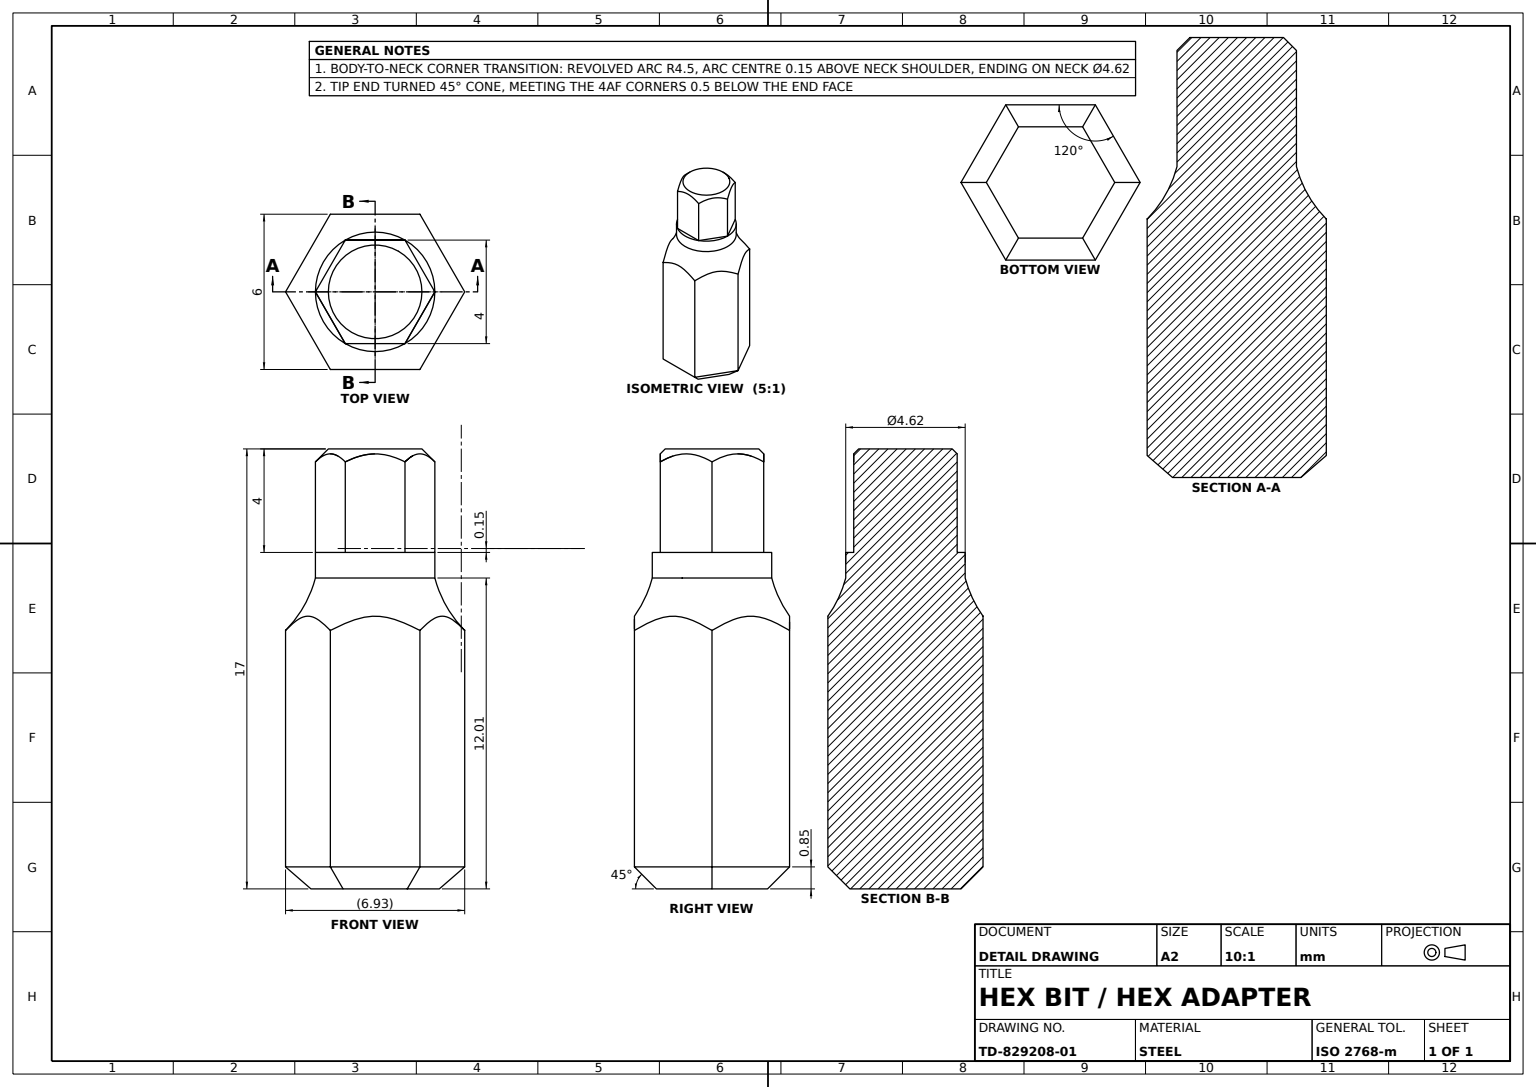
ISO-10303-21;
HEADER;
FILE_DESCRIPTION((''),'2;1');
FILE_NAME('','',(''),(''),'','','');
FILE_SCHEMA(('AUTOMOTIVE_DESIGN'));
ENDSEC;
DATA;
#1=APPLICATION_CONTEXT('');
#2=PRODUCT_CONTEXT('',#1,'mechanical');
#3=PRODUCT('','','',(#2));
#4=PRODUCT_DEFINITION_FORMATION('','',#3);
#5=PRODUCT_DEFINITION_CONTEXT('',#1,'design');
#6=PRODUCT_DEFINITION('','',#4,#5);
#7=PRODUCT_DEFINITION_SHAPE('','',#6);
#8=(LENGTH_UNIT()NAMED_UNIT(*)SI_UNIT(.MILLI.,.METRE.));
#9=(NAMED_UNIT(*)PLANE_ANGLE_UNIT()SI_UNIT($,.RADIAN.));
#10=(NAMED_UNIT(*)SI_UNIT($,.STERADIAN.)SOLID_ANGLE_UNIT());
#11=UNCERTAINTY_MEASURE_WITH_UNIT(LENGTH_MEASURE(1.E-05),#8,'distance_accuracy_value','');
#12=(GEOMETRIC_REPRESENTATION_CONTEXT(3)GLOBAL_UNCERTAINTY_ASSIGNED_CONTEXT((#11))GLOBAL_UNIT_ASSIGNED_CONTEXT((#8,#9,#10))REPRESENTATION_CONTEXT('',''));
#13=CARTESIAN_POINT('',(1.241303,0.,-2.15));
#14=VERTEX_POINT('',#13);
#15=CARTESIAN_POINT('',(2.482606,0.,0.));
#16=VERTEX_POINT('',#15);
#17=CARTESIAN_POINT('',(1.861955,0.,-1.075));
#18=DIRECTION('',(0.5,0.,0.866025404));
#19=VECTOR('',#18,1000.);
#20=LINE('',#17,#19);
#21=EDGE_CURVE('',#14,#16,#20,.T.);
#22=ORIENTED_EDGE('',*,*,#21,.F.);
#23=CARTESIAN_POINT('',(1.732051,0.85,-3.));
#24=VERTEX_POINT('',#23);
#25=DIRECTION('',(0.377964473,0.654653671,-0.654653671));
#26=VECTOR('',#25,1000.);
#27=LINE('',#23,#26);
#28=EDGE_CURVE('',#14,#24,#27,.T.);
#29=ORIENTED_EDGE('',*,*,#28,.T.);
#30=CARTESIAN_POINT('',(3.464102,0.85,0.));
#31=VERTEX_POINT('',#30);
#32=DIRECTION('',(-0.5,0.,-0.866025404));
#33=VECTOR('',#32,1000.);
#34=LINE('',#30,#33);
#35=EDGE_CURVE('',#31,#24,#34,.T.);
#36=ORIENTED_EDGE('',*,*,#35,.F.);
#37=CARTESIAN_POINT('',(2.474358,-0.007143,0.));
#38=DIRECTION('',(-0.755928946,-0.654653671,0.));
#39=VECTOR('',#38,1000.);
#40=LINE('',#37,#39);
#41=EDGE_CURVE('',#31,#16,#40,.T.);
#42=ORIENTED_EDGE('',*,*,#41,.T.);
#43=EDGE_LOOP('',(#22,#29,#36,#42));
#44=FACE_OUTER_BOUND('',#43,.T.);
#45=DIRECTION('',(-0.612372436,0.707106781,0.353553391));
#46=AXIS2_PLACEMENT_3D('',#30,#45,#32);
#47=PLANE('',#46);
#48=ADVANCED_FACE('',(#44),#47,.F.);
#49=CARTESIAN_POINT('',(-2.309401,13.,0.));
#50=VERTEX_POINT('',#49);
#51=CARTESIAN_POINT('',(-1.154701,13.,2.));
#52=VERTEX_POINT('',#51);
#53=LINE('',#49,#19);
#54=EDGE_CURVE('',#50,#52,#53,.T.);
#55=ORIENTED_EDGE('',*,*,#54,.F.);
#56=CARTESIAN_POINT('',(0.,13.,0.));
#57=DIRECTION('',(0.,1.,0.));
#58=DIRECTION('',(-1.,0.,0.));
#59=AXIS2_PLACEMENT_3D('',#56,#57,#58);
#60=CIRCLE('',#59,2.309401);
#61=EDGE_CURVE('',#50,#52,#60,.T.);
#62=ORIENTED_EDGE('',*,*,#61,.T.);
#63=EDGE_LOOP('',(#55,#62));
#64=FACE_OUTER_BOUND('',#63,.T.);
#65=DIRECTION('',(0.,0.,1.));
#66=AXIS2_PLACEMENT_3D('',#56,#57,#65);
#67=PLANE('',#66);
#68=ADVANCED_FACE('',(#64),#67,.T.);
#69=CARTESIAN_POINT('',(1.737869,9.991843,-2.989923));
#70=VERTEX_POINT('',#69);
#71=CARTESIAN_POINT('',(1.732051,9.99905,-3.));
#72=VERTEX_POINT('',#71);
#73=CARTESIAN_POINT('',(1.735928,9.994241,-2.993284));
#74=CARTESIAN_POINT('',(1.733989,9.996643,-2.996643));
#75=B_SPLINE_CURVE_WITH_KNOTS('',3,(#69,#73,#74,#71),.UNSPECIFIED.,.F.,.F.,(4,4),(0.003648524,0.003661967),.UNSPECIFIED.);
#76=EDGE_CURVE('',#70,#72,#75,.T.);
#77=ORIENTED_EDGE('',*,*,#76,.F.);
#78=CARTESIAN_POINT('',(3.458284,9.991843,-0.010077));
#79=VERTEX_POINT('',#78);
#80=CARTESIAN_POINT('',(3.32271,10.128666,-0.244897));
#81=CARTESIAN_POINT('',(3.18628,10.261372,-0.481202));
#82=CARTESIAN_POINT('',(2.972351,10.415848,-0.851738));
#83=CARTESIAN_POINT('',(2.898784,10.459768,-0.979159));
#84=CARTESIAN_POINT('',(2.750308,10.520221,-1.236327));
#85=CARTESIAN_POINT('',(2.67539,10.536765,-1.366089));
#86=CARTESIAN_POINT('',(2.523934,10.537213,-1.628418));
#87=CARTESIAN_POINT('',(2.447185,10.5206,-1.76135));
#88=CARTESIAN_POINT('',(2.298719,10.460482,-2.018502));
#89=CARTESIAN_POINT('',(2.226071,10.417318,-2.144332));
#90=CARTESIAN_POINT('',(2.011174,10.262641,-2.516544));
#91=CARTESIAN_POINT('',(1.873871,10.129099,-2.75436));
#92=B_SPLINE_CURVE_WITH_KNOTS('',3,(#78,#80,#81,#82,#83,#84,#85,#86,#87,#88,#89,#90,#91,#69),.UNSPECIFIED.,.F.,.F.,(4,2,2,2,2,2,4),(0.000000443,0.000909171,0.001363535,0.001817899,0.002272263,0.002726627,0.003635355),.UNSPECIFIED.);
#93=EDGE_CURVE('',#79,#70,#92,.T.);
#94=ORIENTED_EDGE('',*,*,#93,.F.);
#95=CARTESIAN_POINT('',(3.464102,9.99905,0.));
#96=VERTEX_POINT('',#95);
#97=CARTESIAN_POINT('',(3.462163,9.996643,-0.003357));
#98=CARTESIAN_POINT('',(3.460224,9.99424,-0.006716));
#99=B_SPLINE_CURVE_WITH_KNOTS('',3,(#95,#97,#98,#78),.UNSPECIFIED.,.F.,.F.,(4,4),(0.000000939,0.000014451),.UNSPECIFIED.);
#100=EDGE_CURVE('',#96,#79,#99,.T.);
#101=ORIENTED_EDGE('',*,*,#100,.F.);
#102=CARTESIAN_POINT('',(3.464102,17.,0.));
#103=DIRECTION('',(0.,-1.,0.));
#104=VECTOR('',#103,1000.);
#105=LINE('',#102,#104);
#106=EDGE_CURVE('',#96,#31,#105,.T.);
#107=ORIENTED_EDGE('',*,*,#106,.T.);
#108=ORIENTED_EDGE('',*,*,#35,.T.);
#109=CARTESIAN_POINT('',(1.732051,17.,-3.));
#110=LINE('',#109,#104);
#111=EDGE_CURVE('',#72,#24,#110,.T.);
#112=ORIENTED_EDGE('',*,*,#111,.F.);
#113=EDGE_LOOP('',(#77,#94,#101,#107,#108,#112));
#114=FACE_OUTER_BOUND('',#113,.T.);
#115=DIRECTION('',(-0.866025404,0.,0.5));
#116=AXIS2_PLACEMENT_3D('',#102,#115,#18);
#117=PLANE('',#116);
#118=ADVANCED_FACE('',(#114),#117,.F.);
#119=CARTESIAN_POINT('',(1.241303,0.,2.15));
#120=VERTEX_POINT('',#119);
#121=CARTESIAN_POINT('',(-1.241303,0.,2.15));
#122=VERTEX_POINT('',#121);
#123=CARTESIAN_POINT('',(0.,0.,2.15));
#124=VECTOR('',#58,1000.);
#125=LINE('',#123,#124);
#126=EDGE_CURVE('',#120,#122,#125,.T.);
#127=ORIENTED_EDGE('',*,*,#126,.F.);
#128=CARTESIAN_POINT('',(1.732051,0.85,3.));
#129=VERTEX_POINT('',#128);
#130=DIRECTION('',(-0.377964473,-0.654653671,-0.654653671));
#131=VECTOR('',#130,1000.);
#132=LINE('',#128,#131);
#133=EDGE_CURVE('',#129,#120,#132,.T.);
#134=ORIENTED_EDGE('',*,*,#133,.F.);
#135=CARTESIAN_POINT('',(-1.732051,0.85,3.));
#136=VERTEX_POINT('',#135);
#137=DIRECTION('',(1.,0.,0.));
#138=VECTOR('',#137,1000.);
#139=LINE('',#135,#138);
#140=EDGE_CURVE('',#136,#129,#139,.T.);
#141=ORIENTED_EDGE('',*,*,#140,.F.);
#142=DIRECTION('',(0.377964473,-0.654653671,-0.654653671));
#143=VECTOR('',#142,1000.);
#144=LINE('',#135,#143);
#145=EDGE_CURVE('',#136,#122,#144,.T.);
#146=ORIENTED_EDGE('',*,*,#145,.T.);
#147=EDGE_LOOP('',(#127,#134,#141,#146));
#148=FACE_OUTER_BOUND('',#147,.T.);
#149=DIRECTION('',(0.,0.707106781,-0.707106781));
#150=AXIS2_PLACEMENT_3D('',#135,#149,#137);
#151=PLANE('',#150);
#152=ADVANCED_FACE('',(#148),#151,.F.);
#153=CARTESIAN_POINT('',(-1.737869,9.991843,-2.989923));
#154=VERTEX_POINT('',#153);
#155=CARTESIAN_POINT('',(-3.458284,9.991843,-0.010077));
#156=VERTEX_POINT('',#155);
#157=CARTESIAN_POINT('',(-1.873442,10.128666,-2.755103));
#158=CARTESIAN_POINT('',(-2.009873,10.261372,-2.518798));
#159=CARTESIAN_POINT('',(-2.223802,10.415848,-2.148262));
#160=CARTESIAN_POINT('',(-2.297368,10.459768,-2.020841));
#161=CARTESIAN_POINT('',(-2.445845,10.520221,-1.763673));
#162=CARTESIAN_POINT('',(-2.520762,10.536765,-1.633911));
#163=CARTESIAN_POINT('',(-2.672218,10.537213,-1.371582));
#164=CARTESIAN_POINT('',(-2.748967,10.5206,-1.23865));
#165=CARTESIAN_POINT('',(-2.897433,10.460482,-0.981498));
#166=CARTESIAN_POINT('',(-2.970081,10.417318,-0.855668));
#167=CARTESIAN_POINT('',(-3.184978,10.262641,-0.483456));
#168=CARTESIAN_POINT('',(-3.322281,10.129099,-0.24564));
#169=B_SPLINE_CURVE_WITH_KNOTS('',3,(#153,#157,#158,#159,#160,#161,#162,#163,#164,#165,#166,#167,#168,#155),.UNSPECIFIED.,.F.,.F.,(4,2,2,2,2,2,4),(0.000000443,0.000909171,0.001363535,0.001817899,0.002272263,0.002726627,0.003635355),.UNSPECIFIED.);
#170=EDGE_CURVE('',#154,#156,#169,.T.);
#171=ORIENTED_EDGE('',*,*,#170,.T.);
#172=CARTESIAN_POINT('',(-3.458298,9.991843,0.));
#173=VERTEX_POINT('',#172);
#174=CARTESIAN_POINT('',(0.,9.991843,0.));
#175=AXIS2_PLACEMENT_3D('',#174,#57,#58);
#176=CIRCLE('',#175,3.458298);
#177=EDGE_CURVE('',#156,#173,#176,.T.);
#178=ORIENTED_EDGE('',*,*,#177,.T.);
#179=CARTESIAN_POINT('',(-2.309401,12.012039,0.));
#180=VERTEX_POINT('',#179);
#181=CARTESIAN_POINT('',(-6.662857,13.151084,0.));
#182=DIRECTION('',(0.,0.,-1.));
#183=AXIS2_PLACEMENT_3D('',#181,#182,#58);
#184=CIRCLE('',#183,4.5);
#185=EDGE_CURVE('',#180,#173,#184,.T.);
#186=ORIENTED_EDGE('',*,*,#185,.F.);
#187=CARTESIAN_POINT('',(0.,12.012039,-2.309401));
#188=VERTEX_POINT('',#187);
#189=CARTESIAN_POINT('',(0.,12.012039,0.));
#190=AXIS2_PLACEMENT_3D('',#189,#103,#182);
#191=CIRCLE('',#190,2.309401);
#192=EDGE_CURVE('',#180,#188,#191,.T.);
#193=ORIENTED_EDGE('',*,*,#192,.T.);
#194=CARTESIAN_POINT('',(2.309401,12.012039,0.));
#195=VERTEX_POINT('',#194);
#196=EDGE_CURVE('',#188,#195,#191,.T.);
#197=ORIENTED_EDGE('',*,*,#196,.T.);
#198=CARTESIAN_POINT('',(3.458298,9.991843,0.));
#199=VERTEX_POINT('',#198);
#200=CARTESIAN_POINT('',(6.662857,13.151084,0.));
#201=AXIS2_PLACEMENT_3D('',#200,#65,#137);
#202=CIRCLE('',#201,4.5);
#203=EDGE_CURVE('',#195,#199,#202,.T.);
#204=ORIENTED_EDGE('',*,*,#203,.T.);
#205=EDGE_CURVE('',#199,#79,#176,.T.);
#206=ORIENTED_EDGE('',*,*,#205,.T.);
#207=ORIENTED_EDGE('',*,*,#93,.T.);
#208=CARTESIAN_POINT('',(1.720415,9.991843,-3.));
#209=VERTEX_POINT('',#208);
#210=EDGE_CURVE('',#70,#209,#176,.T.);
#211=ORIENTED_EDGE('',*,*,#210,.T.);
#212=CARTESIAN_POINT('',(-1.720415,9.991843,-3.));
#213=VERTEX_POINT('',#212);
#214=CARTESIAN_POINT('',(1.447659,10.129478,-3.));
#215=CARTESIAN_POINT('',(1.172146,10.2633,-3.));
#216=CARTESIAN_POINT('',(0.74373,10.417388,-3.));
#217=CARTESIAN_POINT('',(0.598236,10.460695,-3.));
#218=CARTESIAN_POINT('',(0.298514,10.521144,-3.));
#219=CARTESIAN_POINT('',(0.144906,10.537445,-3.));
#220=CARTESIAN_POINT('',(-0.309493,10.536053,-3.));
#221=CARTESIAN_POINT('',(-0.613618,10.465064,-3.));
#222=CARTESIAN_POINT('',(-1.180792,10.259278,-3.));
#223=CARTESIAN_POINT('',(-1.45149,10.127545,-3.));
#224=B_SPLINE_CURVE_WITH_KNOTS('',3,(#208,#214,#215,#216,#217,#218,#219,#220,#221,#222,#223,#212),.UNSPECIFIED.,.F.,.F.,(4,2,2,2,2,4),(0.004250798,0.005160007,0.005614612,0.006069216,0.006978425,0.007887635),.UNSPECIFIED.);
#225=EDGE_CURVE('',#209,#213,#224,.T.);
#226=ORIENTED_EDGE('',*,*,#225,.T.);
#227=EDGE_CURVE('',#213,#154,#176,.T.);
#228=ORIENTED_EDGE('',*,*,#227,.T.);
#229=EDGE_LOOP('',(#171,#178,#186,#193,#197,#204,#206,#207,#211,#226,#228));
#230=FACE_OUTER_BOUND('',#229,.T.);
#231=CARTESIAN_POINT('',(0.,13.151084,0.));
#232=AXIS2_PLACEMENT_3D('',#231,#57,#58);
#233=TOROIDAL_SURFACE('',#232,6.662857,4.5);
#234=ADVANCED_FACE('',(#230),#233,.F.);
#235=CARTESIAN_POINT('',(-1.720415,9.991843,3.));
#236=VERTEX_POINT('',#235);
#237=CARTESIAN_POINT('',(1.720415,9.991843,3.));
#238=VERTEX_POINT('',#237);
#239=CARTESIAN_POINT('',(-1.447659,10.129478,3.));
#240=CARTESIAN_POINT('',(-1.172146,10.2633,3.));
#241=CARTESIAN_POINT('',(-0.74373,10.417388,3.));
#242=CARTESIAN_POINT('',(-0.598236,10.460695,3.));
#243=CARTESIAN_POINT('',(-0.298514,10.521144,3.));
#244=CARTESIAN_POINT('',(-0.144906,10.537445,3.));
#245=CARTESIAN_POINT('',(0.309493,10.536053,3.));
#246=CARTESIAN_POINT('',(0.613618,10.465064,3.));
#247=CARTESIAN_POINT('',(1.180792,10.259278,3.));
#248=CARTESIAN_POINT('',(1.45149,10.127545,3.));
#249=B_SPLINE_CURVE_WITH_KNOTS('',3,(#235,#239,#240,#241,#242,#243,#244,#245,#246,#247,#248,#237),.UNSPECIFIED.,.F.,.F.,(4,2,2,2,2,4),(0.004250798,0.005160007,0.005614612,0.006069216,0.006978425,0.007887635),.UNSPECIFIED.);
#250=EDGE_CURVE('',#236,#238,#249,.T.);
#251=ORIENTED_EDGE('',*,*,#250,.F.);
#252=CARTESIAN_POINT('',(-1.732051,9.99905,3.));
#253=VERTEX_POINT('',#252);
#254=CARTESIAN_POINT('',(-1.728174,9.996643,3.));
#255=CARTESIAN_POINT('',(-1.724296,9.99424,3.));
#256=B_SPLINE_CURVE_WITH_KNOTS('',3,(#252,#254,#255,#235),.UNSPECIFIED.,.F.,.F.,(4,4),(0.000000813,0.000014325),.UNSPECIFIED.);
#257=EDGE_CURVE('',#253,#236,#256,.T.);
#258=ORIENTED_EDGE('',*,*,#257,.F.);
#259=CARTESIAN_POINT('',(-1.732051,17.,3.));
#260=LINE('',#259,#104);
#261=EDGE_CURVE('',#253,#136,#260,.T.);
#262=ORIENTED_EDGE('',*,*,#261,.T.);
#263=ORIENTED_EDGE('',*,*,#140,.T.);
#264=CARTESIAN_POINT('',(1.732051,9.99905,3.));
#265=VERTEX_POINT('',#264);
#266=CARTESIAN_POINT('',(1.732051,17.,3.));
#267=LINE('',#266,#104);
#268=EDGE_CURVE('',#265,#129,#267,.T.);
#269=ORIENTED_EDGE('',*,*,#268,.F.);
#270=CARTESIAN_POINT('',(1.724296,9.994241,3.));
#271=CARTESIAN_POINT('',(1.728175,9.996643,3.));
#272=B_SPLINE_CURVE_WITH_KNOTS('',3,(#237,#270,#271,#264),.UNSPECIFIED.,.F.,.F.,(4,4),(0.003648403,0.003661846),.UNSPECIFIED.);
#273=EDGE_CURVE('',#238,#265,#272,.T.);
#274=ORIENTED_EDGE('',*,*,#273,.F.);
#275=EDGE_LOOP('',(#251,#258,#262,#263,#269,#274));
#276=FACE_OUTER_BOUND('',#275,.T.);
#277=AXIS2_PLACEMENT_3D('',#259,#182,#58);
#278=PLANE('',#277);
#279=ADVANCED_FACE('',(#276),#278,.F.);
#280=ORIENTED_EDGE('',*,*,#250,.T.);
#281=CARTESIAN_POINT('',(1.737869,9.991843,2.989923));
#282=VERTEX_POINT('',#281);
#283=EDGE_CURVE('',#238,#282,#176,.T.);
#284=ORIENTED_EDGE('',*,*,#283,.T.);
#285=CARTESIAN_POINT('',(3.458284,9.991843,0.010077));
#286=VERTEX_POINT('',#285);
#287=CARTESIAN_POINT('',(1.873442,10.128666,2.755103));
#288=CARTESIAN_POINT('',(2.009873,10.261372,2.518798));
#289=CARTESIAN_POINT('',(2.223802,10.415848,2.148262));
#290=CARTESIAN_POINT('',(2.297368,10.459768,2.020841));
#291=CARTESIAN_POINT('',(2.445845,10.520221,1.763673));
#292=CARTESIAN_POINT('',(2.520762,10.536765,1.633911));
#293=CARTESIAN_POINT('',(2.672218,10.537213,1.371582));
#294=CARTESIAN_POINT('',(2.748967,10.5206,1.23865));
#295=CARTESIAN_POINT('',(2.897433,10.460482,0.981498));
#296=CARTESIAN_POINT('',(2.970081,10.417318,0.855668));
#297=CARTESIAN_POINT('',(3.184978,10.262641,0.483456));
#298=CARTESIAN_POINT('',(3.322281,10.129099,0.24564));
#299=B_SPLINE_CURVE_WITH_KNOTS('',3,(#281,#287,#288,#289,#290,#291,#292,#293,#294,#295,#296,#297,#298,#285),.UNSPECIFIED.,.F.,.F.,(4,2,2,2,2,2,4),(0.000000443,0.000909171,0.001363535,0.001817899,0.002272263,0.002726627,0.003635355),.UNSPECIFIED.);
#300=EDGE_CURVE('',#282,#286,#299,.T.);
#301=ORIENTED_EDGE('',*,*,#300,.T.);
#302=EDGE_CURVE('',#286,#199,#176,.T.);
#303=ORIENTED_EDGE('',*,*,#302,.T.);
#304=ORIENTED_EDGE('',*,*,#203,.F.);
#305=CARTESIAN_POINT('',(0.,12.012039,2.309401));
#306=VERTEX_POINT('',#305);
#307=EDGE_CURVE('',#195,#306,#191,.T.);
#308=ORIENTED_EDGE('',*,*,#307,.T.);
#309=EDGE_CURVE('',#306,#180,#191,.T.);
#310=ORIENTED_EDGE('',*,*,#309,.T.);
#311=ORIENTED_EDGE('',*,*,#185,.T.);
#312=CARTESIAN_POINT('',(-3.458284,9.991843,0.010077));
#313=VERTEX_POINT('',#312);
#314=EDGE_CURVE('',#173,#313,#176,.T.);
#315=ORIENTED_EDGE('',*,*,#314,.T.);
#316=CARTESIAN_POINT('',(-1.737869,9.991843,2.989923));
#317=VERTEX_POINT('',#316);
#318=CARTESIAN_POINT('',(-3.32271,10.128666,0.244897));
#319=CARTESIAN_POINT('',(-3.18628,10.261372,0.481202));
#320=CARTESIAN_POINT('',(-2.972351,10.415848,0.851738));
#321=CARTESIAN_POINT('',(-2.898784,10.459768,0.979159));
#322=CARTESIAN_POINT('',(-2.750308,10.520221,1.236327));
#323=CARTESIAN_POINT('',(-2.67539,10.536765,1.366089));
#324=CARTESIAN_POINT('',(-2.523934,10.537213,1.628418));
#325=CARTESIAN_POINT('',(-2.447185,10.5206,1.76135));
#326=CARTESIAN_POINT('',(-2.298719,10.460482,2.018502));
#327=CARTESIAN_POINT('',(-2.226071,10.417318,2.144332));
#328=CARTESIAN_POINT('',(-2.011174,10.262641,2.516544));
#329=CARTESIAN_POINT('',(-1.873871,10.129099,2.75436));
#330=B_SPLINE_CURVE_WITH_KNOTS('',3,(#312,#318,#319,#320,#321,#322,#323,#324,#325,#326,#327,#328,#329,#316),.UNSPECIFIED.,.F.,.F.,(4,2,2,2,2,2,4),(0.000000443,0.000909171,0.001363535,0.001817899,0.002272263,0.002726627,0.003635355),.UNSPECIFIED.);
#331=EDGE_CURVE('',#313,#317,#330,.T.);
#332=ORIENTED_EDGE('',*,*,#331,.T.);
#333=EDGE_CURVE('',#317,#236,#176,.T.);
#334=ORIENTED_EDGE('',*,*,#333,.T.);
#335=EDGE_LOOP('',(#280,#284,#301,#303,#304,#308,#310,#311,#315,#332,#334));
#336=FACE_OUTER_BOUND('',#335,.T.);
#337=ADVANCED_FACE('',(#336),#233,.F.);
#338=CARTESIAN_POINT('',(1.154701,13.,-2.));
#339=VERTEX_POINT('',#338);
#340=CARTESIAN_POINT('',(0.,13.,-2.309401));
#341=VERTEX_POINT('',#340);
#342=EDGE_CURVE('',#339,#341,#60,.T.);
#343=ORIENTED_EDGE('',*,*,#342,.F.);
#344=CARTESIAN_POINT('',(2.309401,13.,0.));
#345=VERTEX_POINT('',#344);
#346=EDGE_CURVE('',#345,#339,#60,.T.);
#347=ORIENTED_EDGE('',*,*,#346,.F.);
#348=CARTESIAN_POINT('',(1.154701,13.,2.));
#349=VERTEX_POINT('',#348);
#350=EDGE_CURVE('',#349,#345,#60,.T.);
#351=ORIENTED_EDGE('',*,*,#350,.F.);
#352=CARTESIAN_POINT('',(0.,13.,2.309401));
#353=VERTEX_POINT('',#352);
#354=EDGE_CURVE('',#353,#349,#60,.T.);
#355=ORIENTED_EDGE('',*,*,#354,.F.);
#356=CARTESIAN_POINT('',(0.,0.,2.309401));
#357=LINE('',#356,#104);
#358=EDGE_CURVE('',#353,#306,#357,.T.);
#359=ORIENTED_EDGE('',*,*,#358,.T.);
#360=ORIENTED_EDGE('',*,*,#307,.F.);
#361=ORIENTED_EDGE('',*,*,#196,.F.);
#362=CARTESIAN_POINT('',(0.,0.,-2.309401));
#363=LINE('',#362,#104);
#364=EDGE_CURVE('',#341,#188,#363,.T.);
#365=ORIENTED_EDGE('',*,*,#364,.F.);
#366=EDGE_LOOP('',(#343,#347,#351,#355,#359,#360,#361,#365));
#367=FACE_OUTER_BOUND('',#366,.T.);
#368=CARTESIAN_POINT('',(0.,0.,0.));
#369=AXIS2_PLACEMENT_3D('',#368,#103,#182);
#370=CYLINDRICAL_SURFACE('',#369,2.309401);
#371=ADVANCED_FACE('',(#367),#370,.T.);
#372=CARTESIAN_POINT('',(1.809401,17.,0.));
#373=VERTEX_POINT('',#372);
#374=CARTESIAN_POINT('',(2.309401,16.5,0.));
#375=VERTEX_POINT('',#374);
#376=DIRECTION('',(0.707106781,-0.707106781,0.));
#377=VECTOR('',#376,1000.);
#378=LINE('',#374,#377);
#379=EDGE_CURVE('',#373,#375,#378,.T.);
#380=ORIENTED_EDGE('',*,*,#379,.F.);
#381=CARTESIAN_POINT('',(-1.809401,17.,0.));
#382=VERTEX_POINT('',#381);
#383=CARTESIAN_POINT('',(0.,17.,0.));
#384=AXIS2_PLACEMENT_3D('',#383,#57,#58);
#385=CIRCLE('',#384,1.809401);
#386=EDGE_CURVE('',#382,#373,#385,.T.);
#387=ORIENTED_EDGE('',*,*,#386,.F.);
#388=CARTESIAN_POINT('',(-2.309401,16.5,0.));
#389=VERTEX_POINT('',#388);
#390=DIRECTION('',(-0.707106781,-0.707106781,0.));
#391=VECTOR('',#390,1000.);
#392=LINE('',#388,#391);
#393=EDGE_CURVE('',#382,#389,#392,.T.);
#394=ORIENTED_EDGE('',*,*,#393,.T.);
#395=CARTESIAN_POINT('',(-1.154701,16.5,2.));
#396=VERTEX_POINT('',#395);
#397=CARTESIAN_POINT('',(-2.219182,16.590219,0.156264));
#398=CARTESIAN_POINT('',(-2.126928,16.666928,0.316053));
#399=CARTESIAN_POINT('',(-1.983596,16.749129,0.56431));
#400=CARTESIAN_POINT('',(-1.934986,16.770995,0.648507));
#401=CARTESIAN_POINT('',(-1.835708,16.801081,0.82046));
#402=CARTESIAN_POINT('',(-1.784578,16.809182,0.909019));
#403=CARTESIAN_POINT('',(-1.633375,16.809825,1.170912));
#404=CARTESIAN_POINT('',(-1.534293,16.779299,1.342526));
#405=CARTESIAN_POINT('',(-1.338892,16.668565,1.680971));
#406=CARTESIAN_POINT('',(-1.245451,16.590751,1.842815));
#407=B_SPLINE_CURVE_WITH_KNOTS('',3,(#388,#397,#398,#399,#400,#401,#402,#403,#404,#405,#406,#395),.UNSPECIFIED.,.F.,.F.,(4,2,2,2,2,4),(0.000000254,0.000596633,0.000894822,0.001193012,0.00178939,0.002385769),.UNSPECIFIED.);
#408=EDGE_CURVE('',#389,#396,#407,.T.);
#409=ORIENTED_EDGE('',*,*,#408,.T.);
#410=CARTESIAN_POINT('',(1.154701,16.5,2.));
#411=VERTEX_POINT('',#410);
#412=CARTESIAN_POINT('',(-0.975883,16.589409,2.));
#413=CARTESIAN_POINT('',(-0.787603,16.6679,2.));
#414=CARTESIAN_POINT('',(-0.401223,16.777976,2.));
#415=CARTESIAN_POINT('',(-0.20397,16.80926,2.));
#416=CARTESIAN_POINT('',(0.201193,16.809541,2.));
#417=CARTESIAN_POINT('',(0.40141,16.777894,2.));
#418=CARTESIAN_POINT('',(0.786742,16.668174,2.));
#419=CARTESIAN_POINT('',(0.97538,16.58966,2.));
#420=B_SPLINE_CURVE_WITH_KNOTS('',3,(#395,#412,#413,#414,#415,#416,#417,#418,#419,#410),.UNSPECIFIED.,.F.,.F.,(4,2,2,2,4),(0.002943448,0.003545066,0.004146684,0.004748302,0.00534992),.UNSPECIFIED.);
#421=EDGE_CURVE('',#396,#411,#420,.T.);
#422=ORIENTED_EDGE('',*,*,#421,.T.);
#423=CARTESIAN_POINT('',(1.244919,16.590219,1.843736));
#424=CARTESIAN_POINT('',(1.337174,16.666928,1.683947));
#425=CARTESIAN_POINT('',(1.480505,16.749129,1.43569));
#426=CARTESIAN_POINT('',(1.529116,16.770995,1.351493));
#427=CARTESIAN_POINT('',(1.628393,16.801081,1.17954));
#428=CARTESIAN_POINT('',(1.679523,16.809182,1.090981));
#429=CARTESIAN_POINT('',(1.830727,16.809825,0.829088));
#430=CARTESIAN_POINT('',(1.929808,16.779299,0.657474));
#431=CARTESIAN_POINT('',(2.125209,16.668565,0.319029));
#432=CARTESIAN_POINT('',(2.21865,16.590751,0.157185));
#433=B_SPLINE_CURVE_WITH_KNOTS('',3,(#410,#423,#424,#425,#426,#427,#428,#429,#430,#431,#432,#374),.UNSPECIFIED.,.F.,.F.,(4,2,2,2,2,4),(0.000000254,0.000596633,0.000894822,0.001193012,0.00178939,0.002385769),.UNSPECIFIED.);
#434=EDGE_CURVE('',#411,#375,#433,.T.);
#435=ORIENTED_EDGE('',*,*,#434,.T.);
#436=EDGE_LOOP('',(#380,#387,#394,#409,#422,#435));
#437=FACE_OUTER_BOUND('',#436,.T.);
#438=CARTESIAN_POINT('',(0.,16.5,0.));
#439=AXIS2_PLACEMENT_3D('',#438,#103,#137);
#440=CONICAL_SURFACE('',#439,2.309401077,0.785398163);
#441=ADVANCED_FACE('',(#437),#440,.T.);
#442=VECTOR('',#57,1000.);
#443=LINE('',#51,#442);
#444=EDGE_CURVE('',#52,#396,#443,.T.);
#445=ORIENTED_EDGE('',*,*,#444,.T.);
#446=ORIENTED_EDGE('',*,*,#408,.F.);
#447=LINE('',#49,#442);
#448=EDGE_CURVE('',#50,#389,#447,.T.);
#449=ORIENTED_EDGE('',*,*,#448,.F.);
#450=ORIENTED_EDGE('',*,*,#54,.T.);
#451=EDGE_LOOP('',(#445,#446,#449,#450));
#452=FACE_OUTER_BOUND('',#451,.T.);
#453=AXIS2_PLACEMENT_3D('',#49,#115,#18);
#454=PLANE('',#453);
#455=ADVANCED_FACE('',(#452),#454,.T.);
#456=CARTESIAN_POINT('',(-3.464102,9.99905,0.));
#457=VERTEX_POINT('',#456);
#458=CARTESIAN_POINT('',(-3.464102,0.85,0.));
#459=VERTEX_POINT('',#458);
#460=CARTESIAN_POINT('',(-3.464102,17.,0.));
#461=LINE('',#460,#104);
#462=EDGE_CURVE('',#457,#459,#461,.T.);
#463=ORIENTED_EDGE('',*,*,#462,.F.);
#464=CARTESIAN_POINT('',(-3.460224,9.994241,-0.006716));
#465=CARTESIAN_POINT('',(-3.462164,9.996643,-0.003357));
#466=B_SPLINE_CURVE_WITH_KNOTS('',3,(#155,#464,#465,#456),.UNSPECIFIED.,.F.,.F.,(4,4),(0.003648524,0.003661967),.UNSPECIFIED.);
#467=EDGE_CURVE('',#156,#457,#466,.T.);
#468=ORIENTED_EDGE('',*,*,#467,.F.);
#469=ORIENTED_EDGE('',*,*,#170,.F.);
#470=CARTESIAN_POINT('',(-1.732051,9.99905,-3.));
#471=VERTEX_POINT('',#470);
#472=CARTESIAN_POINT('',(-1.733989,9.996643,-2.996643));
#473=CARTESIAN_POINT('',(-1.735928,9.99424,-2.993284));
#474=B_SPLINE_CURVE_WITH_KNOTS('',3,(#470,#472,#473,#153),.UNSPECIFIED.,.F.,.F.,(4,4),(0.000000939,0.000014451),.UNSPECIFIED.);
#475=EDGE_CURVE('',#471,#154,#474,.T.);
#476=ORIENTED_EDGE('',*,*,#475,.F.);
#477=CARTESIAN_POINT('',(-1.732051,0.85,-3.));
#478=VERTEX_POINT('',#477);
#479=CARTESIAN_POINT('',(-1.732051,17.,-3.));
#480=LINE('',#479,#104);
#481=EDGE_CURVE('',#471,#478,#480,.T.);
#482=ORIENTED_EDGE('',*,*,#481,.T.);
#483=DIRECTION('',(-0.5,0.,0.866025404));
#484=VECTOR('',#483,1000.);
#485=LINE('',#477,#484);
#486=EDGE_CURVE('',#478,#459,#485,.T.);
#487=ORIENTED_EDGE('',*,*,#486,.T.);
#488=EDGE_LOOP('',(#463,#468,#469,#476,#482,#487));
#489=FACE_OUTER_BOUND('',#488,.T.);
#490=DIRECTION('',(0.866025404,0.,0.5));
#491=DIRECTION('',(0.5,0.,-0.866025404));
#492=AXIS2_PLACEMENT_3D('',#479,#490,#491);
#493=PLANE('',#492);
#494=ADVANCED_FACE('',(#489),#493,.F.);
#495=ORIENTED_EDGE('',*,*,#434,.F.);
#496=LINE('',#348,#442);
#497=EDGE_CURVE('',#349,#411,#496,.T.);
#498=ORIENTED_EDGE('',*,*,#497,.F.);
#499=VECTOR('',#491,1000.);
#500=LINE('',#348,#499);
#501=EDGE_CURVE('',#349,#345,#500,.T.);
#502=ORIENTED_EDGE('',*,*,#501,.T.);
#503=LINE('',#344,#442);
#504=EDGE_CURVE('',#345,#375,#503,.T.);
#505=ORIENTED_EDGE('',*,*,#504,.T.);
#506=EDGE_LOOP('',(#495,#498,#502,#505));
#507=FACE_OUTER_BOUND('',#506,.T.);
#508=AXIS2_PLACEMENT_3D('',#348,#490,#491);
#509=PLANE('',#508);
#510=ADVANCED_FACE('',(#507),#509,.T.);
#511=EDGE_CURVE('',#52,#353,#60,.T.);
#512=ORIENTED_EDGE('',*,*,#511,.T.);
#513=ORIENTED_EDGE('',*,*,#354,.T.);
#514=LINE('',#51,#138);
#515=EDGE_CURVE('',#52,#349,#514,.T.);
#516=ORIENTED_EDGE('',*,*,#515,.F.);
#517=EDGE_LOOP('',(#512,#513,#516));
#518=FACE_OUTER_BOUND('',#517,.T.);
#519=ADVANCED_FACE('',(#518),#67,.T.);
#520=ORIENTED_EDGE('',*,*,#106,.F.);
#521=CARTESIAN_POINT('',(3.460224,9.994241,0.006716));
#522=CARTESIAN_POINT('',(3.462164,9.996643,0.003357));
#523=B_SPLINE_CURVE_WITH_KNOTS('',3,(#285,#521,#522,#95),.UNSPECIFIED.,.F.,.F.,(4,4),(0.003648524,0.003661967),.UNSPECIFIED.);
#524=EDGE_CURVE('',#286,#96,#523,.T.);
#525=ORIENTED_EDGE('',*,*,#524,.F.);
#526=ORIENTED_EDGE('',*,*,#300,.F.);
#527=CARTESIAN_POINT('',(1.733989,9.996643,2.996643));
#528=CARTESIAN_POINT('',(1.735928,9.99424,2.993284));
#529=B_SPLINE_CURVE_WITH_KNOTS('',3,(#264,#527,#528,#281),.UNSPECIFIED.,.F.,.F.,(4,4),(0.000000939,0.000014451),.UNSPECIFIED.);
#530=EDGE_CURVE('',#265,#282,#529,.T.);
#531=ORIENTED_EDGE('',*,*,#530,.F.);
#532=ORIENTED_EDGE('',*,*,#268,.T.);
#533=LINE('',#128,#499);
#534=EDGE_CURVE('',#129,#31,#533,.T.);
#535=ORIENTED_EDGE('',*,*,#534,.T.);
#536=EDGE_LOOP('',(#520,#525,#526,#531,#532,#535));
#537=FACE_OUTER_BOUND('',#536,.T.);
#538=DIRECTION('',(-0.866025404,0.,-0.5));
#539=AXIS2_PLACEMENT_3D('',#266,#538,#483);
#540=PLANE('',#539);
#541=ADVANCED_FACE('',(#537),#540,.F.);
#542=ORIENTED_EDGE('',*,*,#393,.F.);
#543=EDGE_CURVE('',#373,#382,#385,.T.);
#544=ORIENTED_EDGE('',*,*,#543,.F.);
#545=ORIENTED_EDGE('',*,*,#379,.T.);
#546=CARTESIAN_POINT('',(1.154701,16.5,-2.));
#547=VERTEX_POINT('',#546);
#548=CARTESIAN_POINT('',(2.219182,16.590219,-0.156264));
#549=CARTESIAN_POINT('',(2.126928,16.666928,-0.316053));
#550=CARTESIAN_POINT('',(1.983596,16.749129,-0.56431));
#551=CARTESIAN_POINT('',(1.934986,16.770995,-0.648507));
#552=CARTESIAN_POINT('',(1.835708,16.801081,-0.82046));
#553=CARTESIAN_POINT('',(1.784578,16.809182,-0.909019));
#554=CARTESIAN_POINT('',(1.633375,16.809825,-1.170912));
#555=CARTESIAN_POINT('',(1.534293,16.779299,-1.342526));
#556=CARTESIAN_POINT('',(1.338892,16.668565,-1.680971));
#557=CARTESIAN_POINT('',(1.245451,16.590751,-1.842815));
#558=B_SPLINE_CURVE_WITH_KNOTS('',3,(#374,#548,#549,#550,#551,#552,#553,#554,#555,#556,#557,#546),.UNSPECIFIED.,.F.,.F.,(4,2,2,2,2,4),(0.000000254,0.000596633,0.000894822,0.001193012,0.00178939,0.002385769),.UNSPECIFIED.);
#559=EDGE_CURVE('',#375,#547,#558,.T.);
#560=ORIENTED_EDGE('',*,*,#559,.T.);
#561=CARTESIAN_POINT('',(-1.154701,16.5,-2.));
#562=VERTEX_POINT('',#561);
#563=CARTESIAN_POINT('',(0.975883,16.589409,-2.));
#564=CARTESIAN_POINT('',(0.787603,16.6679,-2.));
#565=CARTESIAN_POINT('',(0.401223,16.777976,-2.));
#566=CARTESIAN_POINT('',(0.20397,16.80926,-2.));
#567=CARTESIAN_POINT('',(-0.201193,16.809541,-2.));
#568=CARTESIAN_POINT('',(-0.40141,16.777894,-2.));
#569=CARTESIAN_POINT('',(-0.786742,16.668174,-2.));
#570=CARTESIAN_POINT('',(-0.97538,16.58966,-2.));
#571=B_SPLINE_CURVE_WITH_KNOTS('',3,(#546,#563,#564,#565,#566,#567,#568,#569,#570,#561),.UNSPECIFIED.,.F.,.F.,(4,2,2,2,4),(0.002943448,0.003545066,0.004146684,0.004748302,0.00534992),.UNSPECIFIED.);
#572=EDGE_CURVE('',#547,#562,#571,.T.);
#573=ORIENTED_EDGE('',*,*,#572,.T.);
#574=CARTESIAN_POINT('',(-1.244919,16.590219,-1.843736));
#575=CARTESIAN_POINT('',(-1.337174,16.666928,-1.683947));
#576=CARTESIAN_POINT('',(-1.480505,16.749129,-1.43569));
#577=CARTESIAN_POINT('',(-1.529116,16.770995,-1.351493));
#578=CARTESIAN_POINT('',(-1.628393,16.801081,-1.17954));
#579=CARTESIAN_POINT('',(-1.679523,16.809182,-1.090981));
#580=CARTESIAN_POINT('',(-1.830727,16.809825,-0.829088));
#581=CARTESIAN_POINT('',(-1.929808,16.779299,-0.657474));
#582=CARTESIAN_POINT('',(-2.125209,16.668565,-0.319029));
#583=CARTESIAN_POINT('',(-2.21865,16.590751,-0.157185));
#584=B_SPLINE_CURVE_WITH_KNOTS('',3,(#561,#574,#575,#576,#577,#578,#579,#580,#581,#582,#583,#388),.UNSPECIFIED.,.F.,.F.,(4,2,2,2,2,4),(0.000000254,0.000596633,0.000894822,0.001193012,0.00178939,0.002385769),.UNSPECIFIED.);
#585=EDGE_CURVE('',#562,#389,#584,.T.);
#586=ORIENTED_EDGE('',*,*,#585,.T.);
#587=EDGE_LOOP('',(#542,#544,#545,#560,#573,#586));
#588=FACE_OUTER_BOUND('',#587,.T.);
#589=ADVANCED_FACE('',(#588),#440,.T.);
#590=CARTESIAN_POINT('',(-1.241303,0.,-2.15));
#591=VERTEX_POINT('',#590);
#592=CARTESIAN_POINT('',(0.,0.,-2.15));
#593=LINE('',#592,#138);
#594=EDGE_CURVE('',#591,#14,#593,.T.);
#595=ORIENTED_EDGE('',*,*,#594,.F.);
#596=DIRECTION('',(-0.377964473,0.654653671,-0.654653671));
#597=VECTOR('',#596,1000.);
#598=LINE('',#477,#597);
#599=EDGE_CURVE('',#591,#478,#598,.T.);
#600=ORIENTED_EDGE('',*,*,#599,.T.);
#601=LINE('',#23,#124);
#602=EDGE_CURVE('',#24,#478,#601,.T.);
#603=ORIENTED_EDGE('',*,*,#602,.F.);
#604=ORIENTED_EDGE('',*,*,#28,.F.);
#605=EDGE_LOOP('',(#595,#600,#603,#604));
#606=FACE_OUTER_BOUND('',#605,.T.);
#607=DIRECTION('',(0.,0.707106781,0.707106781));
#608=AXIS2_PLACEMENT_3D('',#23,#607,#58);
#609=PLANE('',#608);
#610=ADVANCED_FACE('',(#606),#609,.F.);
#611=CARTESIAN_POINT('',(1.728174,9.996643,-3.));
#612=CARTESIAN_POINT('',(1.724296,9.99424,-3.));
#613=B_SPLINE_CURVE_WITH_KNOTS('',3,(#71,#611,#612,#208),.UNSPECIFIED.,.F.,.F.,(4,4),(0.000000813,0.000014325),.UNSPECIFIED.);
#614=EDGE_CURVE('',#72,#209,#613,.T.);
#615=ORIENTED_EDGE('',*,*,#614,.T.);
#616=ORIENTED_EDGE('',*,*,#210,.F.);
#617=ORIENTED_EDGE('',*,*,#76,.T.);
#618=EDGE_LOOP('',(#615,#616,#617));
#619=FACE_OUTER_BOUND('',#618,.T.);
#620=CARTESIAN_POINT('',(0.,19.473541,0.));
#621=AXIS2_PLACEMENT_3D('',#620,#57,#65);
#622=CONICAL_SURFACE('',#621,11.092376237,0.677866184);
#623=ADVANCED_FACE('',(#619),#622,.F.);
#624=ORIENTED_EDGE('',*,*,#205,.F.);
#625=ORIENTED_EDGE('',*,*,#302,.F.);
#626=ORIENTED_EDGE('',*,*,#524,.T.);
#627=ORIENTED_EDGE('',*,*,#100,.T.);
#628=EDGE_LOOP('',(#624,#625,#626,#627));
#629=FACE_OUTER_BOUND('',#628,.T.);
#630=ADVANCED_FACE('',(#629),#622,.F.);
#631=ORIENTED_EDGE('',*,*,#342,.T.);
#632=CARTESIAN_POINT('',(-1.154701,13.,-2.));
#633=VERTEX_POINT('',#632);
#634=EDGE_CURVE('',#341,#633,#60,.T.);
#635=ORIENTED_EDGE('',*,*,#634,.T.);
#636=LINE('',#338,#124);
#637=EDGE_CURVE('',#339,#633,#636,.T.);
#638=ORIENTED_EDGE('',*,*,#637,.F.);
#639=EDGE_LOOP('',(#631,#635,#638));
#640=FACE_OUTER_BOUND('',#639,.T.);
#641=ADVANCED_FACE('',(#640),#67,.T.);
#642=ORIENTED_EDGE('',*,*,#504,.F.);
#643=LINE('',#344,#33);
#644=EDGE_CURVE('',#345,#339,#643,.T.);
#645=ORIENTED_EDGE('',*,*,#644,.T.);
#646=LINE('',#338,#442);
#647=EDGE_CURVE('',#339,#547,#646,.T.);
#648=ORIENTED_EDGE('',*,*,#647,.T.);
#649=ORIENTED_EDGE('',*,*,#559,.F.);
#650=EDGE_LOOP('',(#642,#645,#648,#649));
#651=FACE_OUTER_BOUND('',#650,.T.);
#652=DIRECTION('',(0.866025404,0.,-0.5));
#653=AXIS2_PLACEMENT_3D('',#344,#652,#32);
#654=PLANE('',#653);
#655=ADVANCED_FACE('',(#651),#654,.T.);
#656=ORIENTED_EDGE('',*,*,#543,.T.);
#657=ORIENTED_EDGE('',*,*,#386,.T.);
#658=EDGE_LOOP('',(#656,#657));
#659=FACE_OUTER_BOUND('',#658,.T.);
#660=AXIS2_PLACEMENT_3D('',#383,#57,#65);
#661=PLANE('',#660);
#662=ADVANCED_FACE('',(#659),#661,.T.);
#663=ORIENTED_EDGE('',*,*,#126,.T.);
#664=CARTESIAN_POINT('',(-2.482606,0.,0.));
#665=VERTEX_POINT('',#664);
#666=CARTESIAN_POINT('',(-1.861955,0.,1.075));
#667=LINE('',#666,#33);
#668=EDGE_CURVE('',#122,#665,#667,.T.);
#669=ORIENTED_EDGE('',*,*,#668,.T.);
#670=CARTESIAN_POINT('',(-1.861955,0.,-1.075));
#671=LINE('',#670,#499);
#672=EDGE_CURVE('',#665,#591,#671,.T.);
#673=ORIENTED_EDGE('',*,*,#672,.T.);
#674=ORIENTED_EDGE('',*,*,#594,.T.);
#675=ORIENTED_EDGE('',*,*,#21,.T.);
#676=CARTESIAN_POINT('',(1.861955,0.,1.075));
#677=LINE('',#676,#484);
#678=EDGE_CURVE('',#16,#120,#677,.T.);
#679=ORIENTED_EDGE('',*,*,#678,.T.);
#680=EDGE_LOOP('',(#663,#669,#673,#674,#675,#679));
#681=FACE_OUTER_BOUND('',#680,.T.);
#682=AXIS2_PLACEMENT_3D('',#368,#57,#65);
#683=PLANE('',#682);
#684=ADVANCED_FACE('',(#681),#683,.F.);
#685=ORIENTED_EDGE('',*,*,#599,.F.);
#686=ORIENTED_EDGE('',*,*,#672,.F.);
#687=DIRECTION('',(-0.755928946,0.654653671,0.));
#688=VECTOR('',#687,1000.);
#689=LINE('',#458,#688);
#690=EDGE_CURVE('',#665,#459,#689,.T.);
#691=ORIENTED_EDGE('',*,*,#690,.T.);
#692=ORIENTED_EDGE('',*,*,#486,.F.);
#693=EDGE_LOOP('',(#685,#686,#691,#692));
#694=FACE_OUTER_BOUND('',#693,.T.);
#695=DIRECTION('',(0.612372436,0.707106781,0.353553391));
#696=AXIS2_PLACEMENT_3D('',#477,#695,#483);
#697=PLANE('',#696);
#698=ADVANCED_FACE('',(#694),#697,.F.);
#699=ORIENTED_EDGE('',*,*,#475,.T.);
#700=ORIENTED_EDGE('',*,*,#227,.F.);
#701=CARTESIAN_POINT('',(-1.724296,9.994241,-3.));
#702=CARTESIAN_POINT('',(-1.728175,9.996643,-3.));
#703=B_SPLINE_CURVE_WITH_KNOTS('',3,(#212,#701,#702,#470),.UNSPECIFIED.,.F.,.F.,(4,4),(0.003648403,0.003661846),.UNSPECIFIED.);
#704=EDGE_CURVE('',#213,#471,#703,.T.);
#705=ORIENTED_EDGE('',*,*,#704,.T.);
#706=EDGE_LOOP('',(#699,#700,#705));
#707=FACE_OUTER_BOUND('',#706,.T.);
#708=ADVANCED_FACE('',(#707),#622,.F.);
#709=EDGE_CURVE('',#633,#50,#60,.T.);
#710=ORIENTED_EDGE('',*,*,#709,.T.);
#711=LINE('',#632,#484);
#712=EDGE_CURVE('',#633,#50,#711,.T.);
#713=ORIENTED_EDGE('',*,*,#712,.F.);
#714=EDGE_LOOP('',(#710,#713));
#715=FACE_OUTER_BOUND('',#714,.T.);
#716=ADVANCED_FACE('',(#715),#67,.T.);
#717=CARTESIAN_POINT('',(-3.462163,9.996643,0.003357));
#718=CARTESIAN_POINT('',(-3.460224,9.99424,0.006716));
#719=B_SPLINE_CURVE_WITH_KNOTS('',3,(#456,#717,#718,#312),.UNSPECIFIED.,.F.,.F.,(4,4),(0.000000939,0.000014451),.UNSPECIFIED.);
#720=EDGE_CURVE('',#457,#313,#719,.T.);
#721=ORIENTED_EDGE('',*,*,#720,.F.);
#722=ORIENTED_EDGE('',*,*,#462,.T.);
#723=LINE('',#458,#19);
#724=EDGE_CURVE('',#459,#136,#723,.T.);
#725=ORIENTED_EDGE('',*,*,#724,.T.);
#726=ORIENTED_EDGE('',*,*,#261,.F.);
#727=CARTESIAN_POINT('',(-1.735928,9.994241,2.993284));
#728=CARTESIAN_POINT('',(-1.733989,9.996643,2.996643));
#729=B_SPLINE_CURVE_WITH_KNOTS('',3,(#316,#727,#728,#252),.UNSPECIFIED.,.F.,.F.,(4,4),(0.003648524,0.003661967),.UNSPECIFIED.);
#730=EDGE_CURVE('',#317,#253,#729,.T.);
#731=ORIENTED_EDGE('',*,*,#730,.F.);
#732=ORIENTED_EDGE('',*,*,#331,.F.);
#733=EDGE_LOOP('',(#721,#722,#725,#726,#731,#732));
#734=FACE_OUTER_BOUND('',#733,.T.);
#735=AXIS2_PLACEMENT_3D('',#460,#652,#32);
#736=PLANE('',#735);
#737=ADVANCED_FACE('',(#734),#736,.F.);
#738=ORIENTED_EDGE('',*,*,#346,.T.);
#739=ORIENTED_EDGE('',*,*,#644,.F.);
#740=EDGE_LOOP('',(#738,#739));
#741=FACE_OUTER_BOUND('',#740,.T.);
#742=ADVANCED_FACE('',(#741),#67,.T.);
#743=ORIENTED_EDGE('',*,*,#309,.F.);
#744=ORIENTED_EDGE('',*,*,#358,.F.);
#745=ORIENTED_EDGE('',*,*,#511,.F.);
#746=ORIENTED_EDGE('',*,*,#61,.F.);
#747=ORIENTED_EDGE('',*,*,#709,.F.);
#748=ORIENTED_EDGE('',*,*,#634,.F.);
#749=ORIENTED_EDGE('',*,*,#364,.T.);
#750=ORIENTED_EDGE('',*,*,#192,.F.);
#751=EDGE_LOOP('',(#743,#744,#745,#746,#747,#748,#749,#750));
#752=FACE_OUTER_BOUND('',#751,.T.);
#753=ADVANCED_FACE('',(#752),#370,.T.);
#754=ORIENTED_EDGE('',*,*,#501,.F.);
#755=ORIENTED_EDGE('',*,*,#350,.T.);
#756=EDGE_LOOP('',(#754,#755));
#757=FACE_OUTER_BOUND('',#756,.T.);
#758=ADVANCED_FACE('',(#757),#67,.T.);
#759=ORIENTED_EDGE('',*,*,#444,.F.);
#760=ORIENTED_EDGE('',*,*,#515,.T.);
#761=ORIENTED_EDGE('',*,*,#497,.T.);
#762=ORIENTED_EDGE('',*,*,#421,.F.);
#763=EDGE_LOOP('',(#759,#760,#761,#762));
#764=FACE_OUTER_BOUND('',#763,.T.);
#765=AXIS2_PLACEMENT_3D('',#51,#65,#137);
#766=PLANE('',#765);
#767=ADVANCED_FACE('',(#764),#766,.T.);
#768=ORIENTED_EDGE('',*,*,#111,.T.);
#769=ORIENTED_EDGE('',*,*,#602,.T.);
#770=ORIENTED_EDGE('',*,*,#481,.F.);
#771=ORIENTED_EDGE('',*,*,#704,.F.);
#772=ORIENTED_EDGE('',*,*,#225,.F.);
#773=ORIENTED_EDGE('',*,*,#614,.F.);
#774=EDGE_LOOP('',(#768,#769,#770,#771,#772,#773));
#775=FACE_OUTER_BOUND('',#774,.T.);
#776=AXIS2_PLACEMENT_3D('',#109,#65,#137);
#777=PLANE('',#776);
#778=ADVANCED_FACE('',(#775),#777,.F.);
#779=ORIENTED_EDGE('',*,*,#177,.F.);
#780=ORIENTED_EDGE('',*,*,#467,.T.);
#781=ORIENTED_EDGE('',*,*,#720,.T.);
#782=ORIENTED_EDGE('',*,*,#314,.F.);
#783=EDGE_LOOP('',(#779,#780,#781,#782));
#784=FACE_OUTER_BOUND('',#783,.T.);
#785=ADVANCED_FACE('',(#784),#622,.F.);
#786=ORIENTED_EDGE('',*,*,#257,.T.);
#787=ORIENTED_EDGE('',*,*,#333,.F.);
#788=ORIENTED_EDGE('',*,*,#730,.T.);
#789=EDGE_LOOP('',(#786,#787,#788));
#790=FACE_OUTER_BOUND('',#789,.T.);
#791=ADVANCED_FACE('',(#790),#622,.F.);
#792=ORIENTED_EDGE('',*,*,#690,.F.);
#793=ORIENTED_EDGE('',*,*,#668,.F.);
#794=ORIENTED_EDGE('',*,*,#145,.F.);
#795=ORIENTED_EDGE('',*,*,#724,.F.);
#796=EDGE_LOOP('',(#792,#793,#794,#795));
#797=FACE_OUTER_BOUND('',#796,.T.);
#798=DIRECTION('',(0.612372436,0.707106781,-0.353553391));
#799=AXIS2_PLACEMENT_3D('',#458,#798,#18);
#800=PLANE('',#799);
#801=ADVANCED_FACE('',(#797),#800,.F.);
#802=ORIENTED_EDGE('',*,*,#534,.F.);
#803=ORIENTED_EDGE('',*,*,#133,.T.);
#804=ORIENTED_EDGE('',*,*,#678,.F.);
#805=ORIENTED_EDGE('',*,*,#41,.F.);
#806=EDGE_LOOP('',(#802,#803,#804,#805));
#807=FACE_OUTER_BOUND('',#806,.T.);
#808=DIRECTION('',(-0.612372436,0.707106781,-0.353553391));
#809=AXIS2_PLACEMENT_3D('',#128,#808,#491);
#810=PLANE('',#809);
#811=ADVANCED_FACE('',(#807),#810,.F.);
#812=ORIENTED_EDGE('',*,*,#637,.T.);
#813=LINE('',#632,#442);
#814=EDGE_CURVE('',#633,#562,#813,.T.);
#815=ORIENTED_EDGE('',*,*,#814,.T.);
#816=ORIENTED_EDGE('',*,*,#572,.F.);
#817=ORIENTED_EDGE('',*,*,#647,.F.);
#818=EDGE_LOOP('',(#812,#815,#816,#817));
#819=FACE_OUTER_BOUND('',#818,.T.);
#820=AXIS2_PLACEMENT_3D('',#338,#182,#58);
#821=PLANE('',#820);
#822=ADVANCED_FACE('',(#819),#821,.T.);
#823=ORIENTED_EDGE('',*,*,#283,.F.);
#824=ORIENTED_EDGE('',*,*,#273,.T.);
#825=ORIENTED_EDGE('',*,*,#530,.T.);
#826=EDGE_LOOP('',(#823,#824,#825));
#827=FACE_OUTER_BOUND('',#826,.T.);
#828=ADVANCED_FACE('',(#827),#622,.F.);
#829=ORIENTED_EDGE('',*,*,#712,.T.);
#830=ORIENTED_EDGE('',*,*,#448,.T.);
#831=ORIENTED_EDGE('',*,*,#585,.F.);
#832=ORIENTED_EDGE('',*,*,#814,.F.);
#833=EDGE_LOOP('',(#829,#830,#831,#832));
#834=FACE_OUTER_BOUND('',#833,.T.);
#835=AXIS2_PLACEMENT_3D('',#632,#538,#483);
#836=PLANE('',#835);
#837=ADVANCED_FACE('',(#834),#836,.T.);
#838=CLOSED_SHELL('',(#48,#68,#118,#152,#234,#279,#337,#371,#441,#455,#494,#510,#519,#541,#589,#610,#623,#630,#641,#655,#662,#684,#698,#708,#716,#737,#742,#753,#758,#767,#778,#785,#791,#801,#811,#822,#828,#837));
#839=MANIFOLD_SOLID_BREP('',#838);
#840=ADVANCED_BREP_SHAPE_REPRESENTATION('',(#839),#12);
#841=SHAPE_DEFINITION_REPRESENTATION(#7,#840);
ENDSEC;
END-ISO-10303-21;
